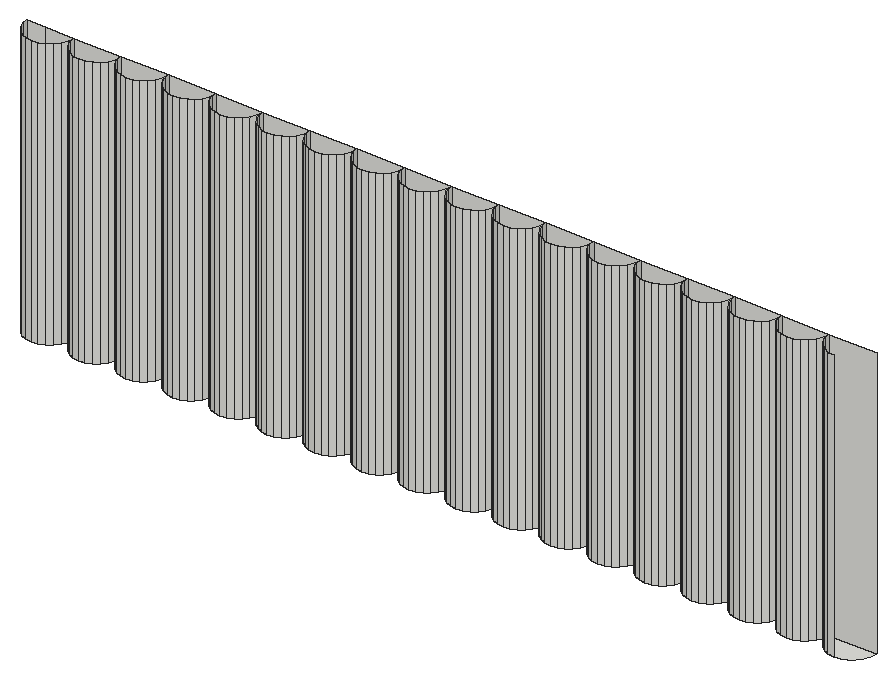
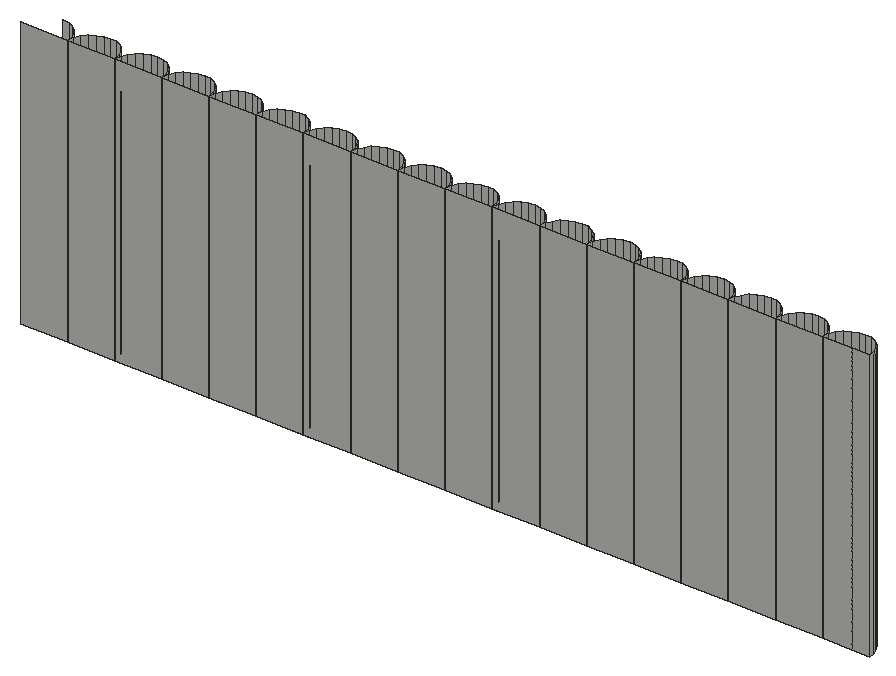
# SketchUp Ruby script. Lengths in inches.
U = 1.inch
M = Sketchup.active_model
def pt(a) = Geom::Point3d.new(a.map { |v| v * U })
def face(e, loops, mat)
  f = e.add_face(loops[0].map { |a| pt(a) })
  loops[1..].each { |l| e.add_face(l.map { |a| pt(a) }).erase! }
  f.material = f.back_material = mat if mat
  f
end
# faces: each face lists its corners as indices into pts; further lists are holes
def faces(e, pts, list, mat = nil) = list.each { |f| face(e, (f[0].is_a?(Array) ? f : [f]).map { |l| l.map { |i| pts[i] } }, mat) }
# xy, xz, yz: faces in a plane at the given z, y or x. An outline is a flat list of corners, or four numbers for a rectangle; further outlines are holes
def ring(l) = l.size == 4 ? [[l[0], l[1]], [l[2], l[1]], [l[2], l[3]], [l[0], l[3]]] : l.each_slice(2).to_a
def flat(e, list, mat, &to3) = list.each { |f| face(e, (f[0].is_a?(Array) ? f : [f]).map { |l| ring(l).map { |u, v| to3.(u, v) } }, mat) }
def xy(e, z, list, mat = nil) = flat(e, list, mat) { |x, y| [x, y, z] }
def xz(e, y, list, mat = nil) = flat(e, list, mat) { |x, z| [x, y, z] }
def yz(e, x, list, mat = nil) = flat(e, list, mat) { |y, z| [x, y, z] }
def lines(e, pts, list) = list.each { |a, b| e.add_line(pt(pts[a]), pt(pts[b])) }
# prism: a flat outline (further loops are holes) pulled along v
def prism(e, loops, v, mat = nil)
  f = face(e, loops, mat); d = Geom::Vector3d.new(v.map { |x| x * U })
  f.pushpull(f.normal.samedirection?(d) ? d.length : -d.length)
end
def box(e, o, s, mat = nil) = prism(e, [[o, [o[0] + s[0], o[1], o[2]], [o[0] + s[0], o[1] + s[1], o[2]], [o[0], o[1] + s[1], o[2]]]], [0, 0, s[2]], mat)
def at(x, y, z, deg = 0) = Geom::Transformation.translation(pt([x, y, z])) * Geom::Transformation.rotation(ORIGIN, Z_AXIS, deg.degrees)
def axes(o, x, y, z) = Geom::Transformation.new([*x, 0, *y, 0, *z, 0, *pt(o).to_a, 1])
def part(name) = M.definitions.add(name)
# library, detail: a bought-in or finely detailed component or shape, given as its bounding box
def library(name, o, s) = part(name).tap { |d| box(d.entities, o, s) }
def detail(e, o, s) = box(e.add_group.entities, o, s)
def put(e, d, t, mat = nil) = e.add_instance(d, t).tap { |i| i.material = mat if mat }
def group(e, t, mat = nil) = e.add_group.tap { |g| g.transformation = t; g.material = mat if mat }.entities
root = M.entities
xy(root,33.18,[[5.77,140.54,5.6,140.5625,5.44,140.63,5.31,140.73,5.2,140.87,5.14,141.03,5.12,141.2,6.43,141.2,6.41,141.03,6.34,140.87,6.24,140.73,6.1,140.63,5.94,140.5625],[7.08,140.54,6.91,140.5625,6.76,140.63,6.62,140.73,6.52,140.87,6.45,141.03,6.43,141.2,7.74,141.2,7.72,141.03,7.65,140.87,7.55,140.73,7.41,140.63,7.25,140.5625],[8.4,140.54,8.23,140.5625,8.07,140.63,7.93,140.73,7.83,140.87,7.76,141.03,7.74,141.2,9.05,141.2,9.03,141.03,8.96,140.87,8.86,140.73,8.72,140.63,8.57,140.5625],[9.71,140.54,9.54,140.5625,9.38,140.63,9.24,140.73,9.14,140.87,9.08,141.03,9.05,141.2,10.37,141.2,10.34,141.03,10.28,140.87,10.17,140.73,10.04,140.63,9.88,140.5625],[11.02,140.54,10.85,140.5625,10.69,140.63,10.56,140.73,10.45,140.87,10.39,141.03,10.37,141.2,11.68,141.2,11.66,141.03,11.59,140.87,11.49,140.73,11.35,140.63,11.19,140.5625],
  [12.33,140.54,12.16,140.5625,12.01,140.63,11.87,140.73,11.77,140.87,11.7,141.03,11.68,141.2,12.99,141.2,12.97,141.03,12.9,140.87,12.8,140.73,12.66,140.63,12.5,140.5625],[13.65,140.54,13.48,140.5625,13.32,140.63,13.18,140.73,13.08,140.87,13.01,141.03,12.99,141.2,14.3,141.2,14.28,141.03,14.21,140.87,14.11,140.73,13.97,140.63,13.82,140.5625],[14.96,140.54,14.79,140.5625,14.63,140.63,14.49,140.73,14.39,140.87,14.33,141.03,14.3,141.2,15.62,141.2,15.59,141.03,15.53,140.87,15.42,140.73,15.29,140.63,15.13,140.5625],[16.27,140.54,16.1,140.5625,15.94,140.63,15.81,140.73,15.7,140.87,15.64,141.03,15.62,141.2,16.93,141.2,16.91,141.03,16.84,140.87,16.74,140.73,16.6,140.63,16.44,140.5625],[17.58,140.54,17.41,140.5625,17.26,140.63,17.12,140.73,17.02,140.87,16.95,141.03,16.93,141.2,18.24,141.2,18.22,141.03,18.15,140.87,18.05,140.73,17.91,140.63,17.75,140.5625],
  [18.9,140.54,18.73,140.5625,18.57,140.63,18.43,140.73,18.33,140.87,18.26,141.03,18.24,141.2,19.55,141.2,19.53,141.03,19.46,140.87,19.36,140.73,19.22,140.63,19.07,140.5625],[20.21,140.54,20.04,140.5625,19.88,140.63,19.74,140.73,19.64,140.87,19.58,141.03,19.55,141.2,20.87,141.2,20.84,141.03,20.78,140.87,20.67,140.73,20.54,140.63,20.38,140.5625],[21.52,140.54,21.35,140.5625,21.19,140.63,21.06,140.73,20.95,140.87,20.89,141.03,20.87,141.2,22.18,141.2,22.16,141.03,22.09,140.87,21.99,140.73,21.85,140.63,21.69,140.5625],[22.83,140.54,22.66,140.5625,22.51,140.63,22.37,140.73,22.27,140.87,22.2,141.03,22.18,141.2,23.49,141.2,23.47,141.03,23.4,140.87,23.3,140.73,23.16,140.63,23,140.5625],[24.15,140.54,23.98,140.5625,23.82,140.63,23.68,140.73,23.58,140.87,23.51,141.03,23.49,141.2,24.8,141.2,24.78,141.03,24.71,140.87,24.61,140.73,24.47,140.63,24.32,140.5625],
  [25.46,140.54,25.29,140.5625,25.13,140.63,24.99,140.73,24.89,140.87,24.83,141.03,24.8,141.2,26.12,141.2,26.09,141.03,26.03,140.87,25.92,140.73,25.79,140.63,25.63,140.5625],[26.77,140.54,26.6,140.5625,26.44,140.63,26.31,140.73,26.2,140.87,26.14,141.03,26.12,141.2,27.43,141.2,27.41,141.03,27.34,140.87,27.24,140.73,27.1,140.63,26.94,140.5625],[28.08,140.54,27.91,140.5625,27.76,140.63,27.62,140.73,27.52,140.87,27.45,141.03,27.43,141.2,28.74,141.2,28.72,141.03,28.65,140.87,28.55,140.73,28.41,140.63,28.25,140.5625]])
xz(root,141.2,[[5.12,33.18,5.62,40.6875],[5.62,33.18,6.43,40.6875],[6.43,33.18,7.74,40.6875],[7.74,33.18,9.05,40.6875],[9.05,33.18,10.37,40.6875],
  [10.37,33.18,11.68,40.6875],[11.68,33.18,12.99,40.6875],[12.99,33.18,14.3,40.6875],[14.3,33.18,15.62,40.6875],[15.62,33.18,16.93,40.6875],
  [16.93,33.18,18.24,40.6875],[18.24,33.18,19.55,40.6875],[19.55,33.18,20.87,40.6875],[20.87,33.18,22.18,40.6875],[22.18,33.18,23.49,40.6875],
  [23.49,33.18,24.8,40.6875],[24.8,33.18,26.12,40.6875],[26.12,33.18,27.43,40.6875],[27.43,33.18,28.74,40.6875]])
p = [[5.6,140.5625,33.18],[5.77,140.54,33.18],[5.77,140.54,40.6875],[5.6,140.5625,40.6875],[5.94,140.5625,33.18],[5.94,140.5625,40.6875],
  [6.91,140.5625,33.18],[7.08,140.54,33.18],[7.08,140.54,40.6875],[6.91,140.5625,40.6875],[7.25,140.5625,33.18],[7.25,140.5625,40.6875],
  [8.23,140.5625,33.18],[8.4,140.54,33.18],[8.4,140.54,40.6875],[8.23,140.5625,40.6875],[8.57,140.5625,33.18],[8.57,140.5625,40.6875],
  [9.54,140.5625,33.18],[9.71,140.54,33.18],[9.71,140.54,40.6875],[9.54,140.5625,40.6875],[9.88,140.5625,33.18],[9.88,140.5625,40.6875],
  [10.85,140.5625,33.18],[11.02,140.54,33.18],[11.02,140.54,40.6875],[10.85,140.5625,40.6875],[11.19,140.5625,33.18],[11.19,140.5625,40.6875],
  [12.16,140.5625,33.18],[12.33,140.54,33.18],[12.33,140.54,40.6875],[12.16,140.5625,40.6875],[12.5,140.5625,33.18],[12.5,140.5625,40.6875],
  [13.48,140.5625,33.18],[13.65,140.54,33.18],[13.65,140.54,40.6875],[13.48,140.5625,40.6875],[13.82,140.5625,33.18],[13.82,140.5625,40.6875],
  [14.79,140.5625,33.18],[14.96,140.54,33.18],[14.96,140.54,40.6875],[14.79,140.5625,40.6875],[15.13,140.5625,33.18],[15.13,140.5625,40.6875],
  [16.1,140.5625,33.18],[16.27,140.54,33.18],[16.27,140.54,40.6875],[16.1,140.5625,40.6875],[16.44,140.5625,33.18],[16.44,140.5625,40.6875],
  [17.41,140.5625,33.18],[17.58,140.54,33.18],[17.58,140.54,40.6875],[17.41,140.5625,40.6875],[17.75,140.5625,33.18],[17.75,140.5625,40.6875],
  [18.73,140.5625,33.18],[18.9,140.54,33.18],[18.9,140.54,40.6875],[18.73,140.5625,40.6875],[19.07,140.5625,33.18],[19.07,140.5625,40.6875],
  [20.04,140.5625,33.18],[20.21,140.54,33.18],[20.21,140.54,40.6875],[20.04,140.5625,40.6875],[20.38,140.5625,33.18],[20.38,140.5625,40.6875],
  [21.35,140.5625,33.18],[21.52,140.54,33.18],[21.52,140.54,40.6875],[21.35,140.5625,40.6875],[21.69,140.5625,33.18],[21.69,140.5625,40.6875],
  [22.66,140.5625,33.18],[22.83,140.54,33.18],[22.83,140.54,40.6875],[22.66,140.5625,40.6875],[23,140.5625,33.18],[23,140.5625,40.6875],
  [23.98,140.5625,33.18],[24.15,140.54,33.18],[24.15,140.54,40.6875],[23.98,140.5625,40.6875],[24.32,140.5625,33.18],[24.32,140.5625,40.6875],
  [25.29,140.5625,33.18],[25.46,140.54,33.18],[25.46,140.54,40.6875],[25.29,140.5625,40.6875],[25.63,140.5625,33.18],[25.63,140.5625,40.6875],
  [26.6,140.5625,33.18],[26.77,140.54,33.18],[26.77,140.54,40.6875],[26.6,140.5625,40.6875],[26.94,140.5625,33.18],[26.94,140.5625,40.6875],
  [27.91,140.5625,33.18],[28.08,140.54,33.18],[28.08,140.54,40.6875],[27.91,140.5625,40.6875],[5.31,140.73,33.18],[5.44,140.63,33.18],
  [5.44,140.63,40.6875],[5.31,140.73,40.6875],[6.1,140.63,33.18],[6.1,140.63,40.6875],[6.24,140.73,33.18],[6.24,140.73,40.6875],
  [6.62,140.73,33.18],[6.76,140.63,33.18],[6.76,140.63,40.6875],[6.62,140.73,40.6875],[7.41,140.63,33.18],[7.41,140.63,40.6875],
  [7.55,140.73,33.18],[7.55,140.73,40.6875],[7.93,140.73,33.18],[8.07,140.63,33.18],[8.07,140.63,40.6875],[7.93,140.73,40.6875],
  [8.72,140.63,33.18],[8.72,140.63,40.6875],[8.86,140.73,33.18],[8.86,140.73,40.6875],[9.24,140.73,33.18],[9.38,140.63,33.18],
  [9.38,140.63,40.6875],[9.24,140.73,40.6875],[10.04,140.63,33.18],[10.04,140.63,40.6875],[10.17,140.73,33.18],[10.17,140.73,40.6875],
  [10.56,140.73,33.18],[10.69,140.63,33.18],[10.69,140.63,40.6875],[10.56,140.73,40.6875],[11.35,140.63,33.18],[11.35,140.63,40.6875],
  [11.49,140.73,33.18],[11.49,140.73,40.6875],[11.87,140.73,33.18],[12.01,140.63,33.18],[12.01,140.63,40.6875],[11.87,140.73,40.6875],
  [12.66,140.63,33.18],[12.66,140.63,40.6875],[12.8,140.73,33.18],[12.8,140.73,40.6875],[13.18,140.73,33.18],[13.32,140.63,33.18],
  [13.32,140.63,40.6875],[13.18,140.73,40.6875],[13.97,140.63,33.18],[13.97,140.63,40.6875],[14.11,140.73,33.18],[14.11,140.73,40.6875],
  [14.49,140.73,33.18],[14.63,140.63,33.18],[14.63,140.63,40.6875],[14.49,140.73,40.6875],[15.29,140.63,33.18],[15.29,140.63,40.6875],
  [15.42,140.73,33.18],[15.42,140.73,40.6875],[15.81,140.73,33.18],[15.94,140.63,33.18],[15.94,140.63,40.6875],[15.81,140.73,40.6875],
  [16.6,140.63,33.18],[16.6,140.63,40.6875],[16.74,140.73,33.18],[16.74,140.73,40.6875],[17.12,140.73,33.18],[17.26,140.63,33.18],
  [17.26,140.63,40.6875],[17.12,140.73,40.6875],[17.91,140.63,33.18],[17.91,140.63,40.6875],[18.05,140.73,33.18],[18.05,140.73,40.6875],
  [18.43,140.73,33.18],[18.57,140.63,33.18],[18.57,140.63,40.6875],[18.43,140.73,40.6875],[19.22,140.63,33.18],[19.22,140.63,40.6875],
  [19.36,140.73,33.18],[19.36,140.73,40.6875],[19.74,140.73,33.18],[19.88,140.63,33.18],[19.88,140.63,40.6875],[19.74,140.73,40.6875],
  [20.54,140.63,33.18],[20.54,140.63,40.6875],[20.67,140.73,33.18],[20.67,140.73,40.6875],[21.06,140.73,33.18],[21.19,140.63,33.18],
  [21.19,140.63,40.6875],[21.06,140.73,40.6875],[21.85,140.63,33.18],[21.85,140.63,40.6875],[21.99,140.73,33.18],[21.99,140.73,40.6875],
  [22.37,140.73,33.18],[22.51,140.63,33.18],[22.51,140.63,40.6875],[22.37,140.73,40.6875],[23.16,140.63,33.18],[23.16,140.63,40.6875],
  [23.3,140.73,33.18],[23.3,140.73,40.6875],[23.68,140.73,33.18],[23.82,140.63,33.18],[23.82,140.63,40.6875],[23.68,140.73,40.6875],
  [24.47,140.63,33.18],[24.47,140.63,40.6875],[24.61,140.73,33.18],[24.61,140.73,40.6875],[24.99,140.73,33.18],[25.13,140.63,33.18],
  [25.13,140.63,40.6875],[24.99,140.73,40.6875],[25.79,140.63,33.18],[25.79,140.63,40.6875],[25.92,140.73,33.18],[25.92,140.73,40.6875],
  [26.31,140.73,33.18],[26.44,140.63,33.18],[26.44,140.63,40.6875],[26.31,140.73,40.6875],[27.1,140.63,33.18],[27.1,140.63,40.6875],
  [27.24,140.73,33.18],[27.24,140.73,40.6875],[27.62,140.73,33.18],[27.76,140.63,33.18],[27.76,140.63,40.6875],[27.62,140.73,40.6875],
  [5.2,140.87,33.18],[5.2,140.87,40.6875],[6.34,140.87,33.18],[6.34,140.87,40.6875],[6.52,140.87,33.18],[6.52,140.87,40.6875],
  [7.65,140.87,33.18],[7.65,140.87,40.6875],[7.83,140.87,33.18],[7.83,140.87,40.6875],[8.96,140.87,33.18],[8.96,140.87,40.6875],
  [9.14,140.87,33.18],[9.14,140.87,40.6875],[10.28,140.87,33.18],[10.28,140.87,40.6875],[10.45,140.87,33.18],[10.45,140.87,40.6875],
  [11.59,140.87,33.18],[11.59,140.87,40.6875],[11.77,140.87,33.18],[11.77,140.87,40.6875],[12.9,140.87,33.18],[12.9,140.87,40.6875],
  [13.08,140.87,33.18],[13.08,140.87,40.6875],[14.21,140.87,33.18],[14.21,140.87,40.6875],[14.39,140.87,33.18],[14.39,140.87,40.6875],
  [15.53,140.87,33.18],[15.53,140.87,40.6875],[15.7,140.87,33.18],[15.7,140.87,40.6875],[16.84,140.87,33.18],[16.84,140.87,40.6875],
  [17.02,140.87,33.18],[17.02,140.87,40.6875],[18.15,140.87,33.18],[18.15,140.87,40.6875],[18.33,140.87,33.18],[18.33,140.87,40.6875],
  [19.46,140.87,33.18],[19.46,140.87,40.6875],[19.64,140.87,33.18],[19.64,140.87,40.6875],[20.78,140.87,33.18],[20.78,140.87,40.6875],
  [20.95,140.87,33.18],[20.95,140.87,40.6875],[22.09,140.87,33.18],[22.09,140.87,40.6875],[22.27,140.87,33.18],[22.27,140.87,40.6875],
  [23.4,140.87,33.18],[23.4,140.87,40.6875],[23.58,140.87,33.18],[23.58,140.87,40.6875],[24.71,140.87,33.18],[24.71,140.87,40.6875],
  [24.89,140.87,33.18],[24.89,140.87,40.6875],[26.03,140.87,33.18],[26.03,140.87,40.6875],[26.2,140.87,33.18],[26.2,140.87,40.6875],
  [27.34,140.87,33.18],[27.34,140.87,40.6875],[27.52,140.87,33.18],[27.52,140.87,40.6875],[5.14,141.03,33.18],[5.14,141.03,40.6875],
  [6.41,141.03,33.18],[6.41,141.03,40.6875],[6.45,141.03,33.18],[6.45,141.03,40.6875],[7.72,141.03,33.18],[7.72,141.03,40.6875],
  [7.76,141.03,33.18],[7.76,141.03,40.6875],[9.03,141.03,33.18],[9.03,141.03,40.6875],[9.08,141.03,33.18],[9.08,141.03,40.6875],
  [10.34,141.03,33.18],[10.34,141.03,40.6875],[10.39,141.03,33.18],[10.39,141.03,40.6875],[11.66,141.03,33.18],[11.66,141.03,40.6875],
  [11.7,141.03,33.18],[11.7,141.03,40.6875],[12.97,141.03,33.18],[12.97,141.03,40.6875],[13.01,141.03,33.18],[13.01,141.03,40.6875],
  [14.28,141.03,33.18],[14.28,141.03,40.6875],[14.33,141.03,33.18],[14.33,141.03,40.6875],[15.59,141.03,33.18],[15.59,141.03,40.6875],
  [15.64,141.03,33.18],[15.64,141.03,40.6875],[16.91,141.03,33.18],[16.91,141.03,40.6875],[16.95,141.03,33.18],[16.95,141.03,40.6875],
  [18.22,141.03,33.18],[18.22,141.03,40.6875],[18.26,141.03,33.18],[18.26,141.03,40.6875],[19.53,141.03,33.18],[19.53,141.03,40.6875],
  [19.58,141.03,33.18],[19.58,141.03,40.6875],[20.84,141.03,33.18],[20.84,141.03,40.6875],[20.89,141.03,33.18],[20.89,141.03,40.6875],
  [22.16,141.03,33.18],[22.16,141.03,40.6875],[22.2,141.03,33.18],[22.2,141.03,40.6875],[23.47,141.03,33.18],[23.47,141.03,40.6875],
  [23.51,141.03,33.18],[23.51,141.03,40.6875],[24.78,141.03,33.18],[24.78,141.03,40.6875],[24.83,141.03,33.18],[24.83,141.03,40.6875],
  [26.09,141.03,33.18],[26.09,141.03,40.6875],[26.14,141.03,33.18],[26.14,141.03,40.6875],[27.41,141.03,33.18],[27.41,141.03,40.6875],
  [27.45,141.03,33.18],[27.45,141.03,40.6875],[5.12,141.2,33.18],[5.12,141.2,40.6875],[6.43,141.2,33.18],[6.43,141.2,40.6875],
  [7.74,141.2,33.18],[7.74,141.2,40.6875],[9.05,141.2,33.18],[9.05,141.2,40.6875],[10.37,141.2,33.18],[10.37,141.2,40.6875],
  [11.68,141.2,33.18],[11.68,141.2,40.6875],[12.99,141.2,33.18],[12.99,141.2,40.6875],[14.3,141.2,33.18],[14.3,141.2,40.6875],
  [15.62,141.2,33.18],[15.62,141.2,40.6875],[16.93,141.2,33.18],[16.93,141.2,40.6875],[18.24,141.2,33.18],[18.24,141.2,40.6875],
  [19.55,141.2,33.18],[19.55,141.2,40.6875],[20.87,141.2,33.18],[20.87,141.2,40.6875],[22.18,141.2,33.18],[22.18,141.2,40.6875],
  [23.49,141.2,33.18],[23.49,141.2,40.6875],[24.8,141.2,33.18],[24.8,141.2,40.6875],[26.12,141.2,33.18],[26.12,141.2,40.6875],
  [27.43,141.2,33.18],[27.43,141.2,40.6875]]
faces(root,p,[[0,1,2,3],[1,4,5,2],[6,7,8,9],[7,10,11,8],[12,13,14,15],[13,16,17,14],[18,19,20,21],[19,22,23,20],
  [24,25,26,27],[25,28,29,26],[30,31,32,33],[31,34,35,32],[36,37,38,39],[37,40,41,38],[42,43,44,45],[43,46,47,44],
  [48,49,50,51],[49,52,53,50],[54,55,56,57],[55,58,59,56],[60,61,62,63],[61,64,65,62],[66,67,68,69],[67,70,71,68],
  [72,73,74,75],[73,76,77,74],[78,79,80,81],[79,82,83,80],[84,85,86,87],[85,88,89,86],[90,91,92,93],[91,94,95,92],
  [96,97,98,99],[97,100,101,98],[102,103,104,105],[106,107,108,109],[107,0,3,108],[4,110,111,5],[110,112,113,111],[114,115,116,117],
  [115,6,9,116],[10,118,119,11],[118,120,121,119],[122,123,124,125],[123,12,15,124],[16,126,127,17],[126,128,129,127],[130,131,132,133],
  [131,18,21,132],[22,134,135,23],[134,136,137,135],[138,139,140,141],[139,24,27,140],[28,142,143,29],[142,144,145,143],[146,147,148,149],
  [147,30,33,148],[34,150,151,35],[150,152,153,151],[154,155,156,157],[155,36,39,156],[40,158,159,41],[158,160,161,159],[162,163,164,165],
  [163,42,45,164],[46,166,167,47],[166,168,169,167],[170,171,172,173],[171,48,51,172],[52,174,175,53],[174,176,177,175],[178,179,180,181],
  [179,54,57,180],[58,182,183,59],[182,184,185,183],[186,187,188,189],[187,60,63,188],[64,190,191,65],[190,192,193,191],[194,195,196,197],
  [195,66,69,196],[70,198,199,71],[198,200,201,199],[202,203,204,205],[203,72,75,204],[76,206,207,77],[206,208,209,207],[210,211,212,213],
  [211,78,81,212],[82,214,215,83],[214,216,217,215],[218,219,220,221],[219,84,87,220],[88,222,223,89],[222,224,225,223],[226,227,228,229],
  [227,90,93,228],[94,230,231,95],[230,232,233,231],[234,235,236,237],[235,96,99,236],[100,238,239,101],[238,240,241,239],[242,243,244,245],
  [243,102,105,244],[246,106,109,247],[112,248,249,113],[250,114,117,251],[120,252,253,121],[254,122,125,255],[128,256,257,129],[258,130,133,259],
  [136,260,261,137],[262,138,141,263],[144,264,265,145],[266,146,149,267],[152,268,269,153],[270,154,157,271],[160,272,273,161],[274,162,165,275],
  [168,276,277,169],[278,170,173,279],[176,280,281,177],[282,178,181,283],[184,284,285,185],[286,186,189,287],[192,288,289,193],[290,194,197,291],
  [200,292,293,201],[294,202,205,295],[208,296,297,209],[298,210,213,299],[216,300,301,217],[302,218,221,303],[224,304,305,225],[306,226,229,307],
  [232,308,309,233],[310,234,237,311],[240,312,313,241],[314,242,245,315],[316,246,247,317],[248,318,319,249],[320,250,251,321],[252,322,323,253],
  [324,254,255,325],[256,326,327,257],[328,258,259,329],[260,330,331,261],[332,262,263,333],[264,334,335,265],[336,266,267,337],[268,338,339,269],
  [340,270,271,341],[272,342,343,273],[344,274,275,345],[276,346,347,277],[348,278,279,349],[280,350,351,281],[352,282,283,353],[284,354,355,285],
  [356,286,287,357],[288,358,359,289],[360,290,291,361],[292,362,363,293],[364,294,295,365],[296,366,367,297],[368,298,299,369],[300,370,371,301],
  [372,302,303,373],[304,374,375,305],[376,306,307,377],[308,378,379,309],[380,310,311,381],[312,382,383,313],[384,314,315,385],[386,316,317,387],
  [318,388,389,319],[388,320,321,389],[322,390,391,323],[390,324,325,391],[326,392,393,327],[392,328,329,393],[330,394,395,331],[394,332,333,395],
  [334,396,397,335],[396,336,337,397],[338,398,399,339],[398,340,341,399],[342,400,401,343],[400,344,345,401],[346,402,403,347],[402,348,349,403],
  [350,404,405,351],[404,352,353,405],[354,406,407,355],[406,356,357,407],[358,408,409,359],[408,360,361,409],[362,410,411,363],[410,364,365,411],
  [366,412,413,367],[412,368,369,413],[370,414,415,371],[414,372,373,415],[374,416,417,375],[416,376,377,417],[378,418,419,379],[418,380,381,419],
  [382,420,421,383],[420,384,385,421]])
